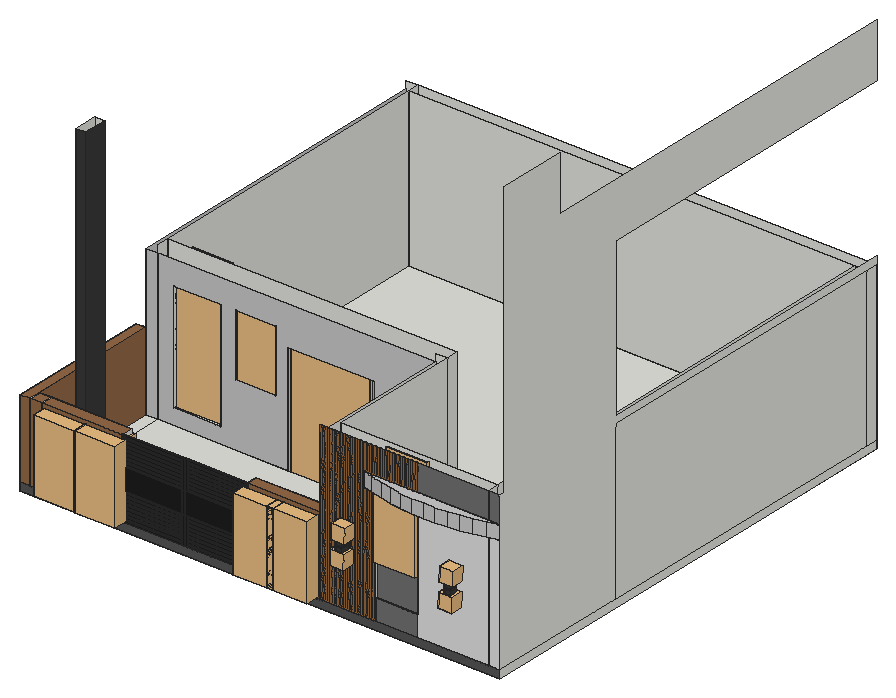
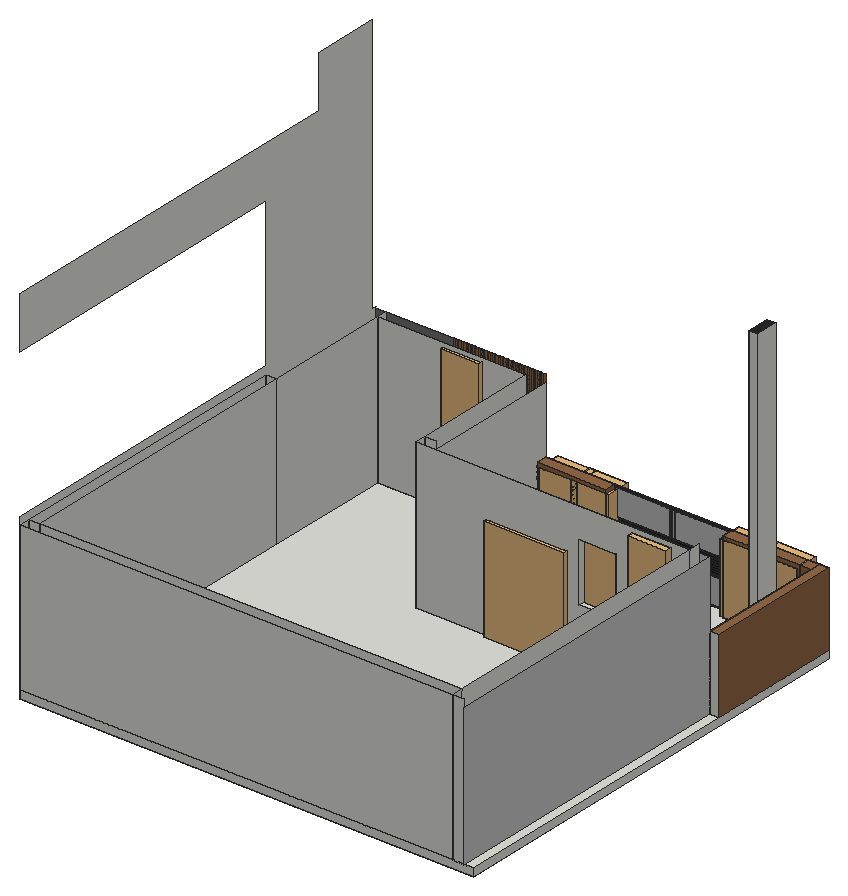
# SketchUp Ruby script. Lengths in inches.
U = 1.inch
M = Sketchup.active_model
def pt(a) = Geom::Point3d.new(a.map { |v| v * U })
def face(e, loops, mat)
  f = e.add_face(loops[0].map { |a| pt(a) })
  loops[1..].each { |l| e.add_face(l.map { |a| pt(a) }).erase! }
  f.material = f.back_material = mat if mat
  f
end
# faces: each face lists its corners as indices into pts; further lists are holes
def faces(e, pts, list, mat = nil) = list.each { |f| face(e, (f[0].is_a?(Array) ? f : [f]).map { |l| l.map { |i| pts[i] } }, mat) }
# xy, xz, yz: faces in a plane at the given z, y or x. An outline is a flat list of corners, or four numbers for a rectangle; further outlines are holes
def ring(l) = l.size == 4 ? [[l[0], l[1]], [l[2], l[1]], [l[2], l[3]], [l[0], l[3]]] : l.each_slice(2).to_a
def flat(e, list, mat, &to3) = list.each { |f| face(e, (f[0].is_a?(Array) ? f : [f]).map { |l| ring(l).map { |u, v| to3.(u, v) } }, mat) }
def xy(e, z, list, mat = nil) = flat(e, list, mat) { |x, y| [x, y, z] }
def xz(e, y, list, mat = nil) = flat(e, list, mat) { |x, z| [x, y, z] }
def yz(e, x, list, mat = nil) = flat(e, list, mat) { |y, z| [x, y, z] }
def lines(e, pts, list) = list.each { |a, b| e.add_line(pt(pts[a]), pt(pts[b])) }
# prism: a flat outline (further loops are holes) pulled along v
def prism(e, loops, v, mat = nil)
  f = face(e, loops, mat); d = Geom::Vector3d.new(v.map { |x| x * U })
  f.pushpull(f.normal.samedirection?(d) ? d.length : -d.length)
end
def box(e, o, s, mat = nil) = prism(e, [[o, [o[0] + s[0], o[1], o[2]], [o[0] + s[0], o[1] + s[1], o[2]], [o[0], o[1] + s[1], o[2]]]], [0, 0, s[2]], mat)
def at(x, y, z, deg = 0) = Geom::Transformation.translation(pt([x, y, z])) * Geom::Transformation.rotation(ORIGIN, Z_AXIS, deg.degrees)
def axes(o, x, y, z) = Geom::Transformation.new([*x, 0, *y, 0, *z, 0, *pt(o).to_a, 1])
def part(name) = M.definitions.add(name)
# library, detail: a bought-in or finely detailed component or shape, given as its bounding box
def library(name, o, s) = part(name).tap { |d| box(d.entities, o, s) }
def detail(e, o, s) = box(e.add_group.entities, o, s)
def put(e, d, t, mat = nil) = e.add_instance(d, t).tap { |i| i.material = mat if mat }
def group(e, t, mat = nil) = e.add_group.tap { |g| g.transformation = t; g.material = mat if mat }.entities
root = M.entities
M.materials.add("11.free-metal-textures").color = [58, 58, 58]
M.materials.add("Color_008").color = [30, 30, 30]
M.materials.add("[0055_LightGoldenrodYellow]").color = [250, 250, 210]
M.materials.add("[0111_SlateGray]1").color = [112, 128, 144]
M.materials.add("[0117_GhostWhite]").color = [248, 248, 255]
M.materials.add("[0131_Silver]1").color = [192, 192, 192]
M.materials.add("[0134_DimGray]").color = [105, 105, 105]
M.materials.add("[Brick Antique 01]").color = [147, 105, 71]
M.materials.add("[Cladding Stucco White]").color = [200, 200, 200]
M.materials.add("[Color M01]").color = [226, 226, 226]
M.materials.add("[Color M05]").color = [114, 114, 114]
M.materials.add("[Color M06]").color = [86, 86, 86]
M.materials.add("[Color M07]").color = [58, 58, 58]
M.materials.add("[Wood Floor]").color = [155, 105, 61]
M.materials.add("images").color = [124, 124, 124]
c1 = library("Door 243 053",[-21.6,-2.79,-0.07],[43.2,5.58,82.64])
c2 = part("Gate slat")
box(c2.entities,[0,0,-2.03],[1.97,0.97,40.94])
c3 = part("Gate frame upright")
box(c3.entities,[0,0,0],[1.9,0.97,93.54])
c4 = part("Gate slat \#1")
box(c4.entities,[2.95,0,-2.03],[0.99,0.97,40.94])
c5 = part("Slatted gate panel")
p = [[42.85,0.97,43.31],[42.85,0.97,44.29]]
lines(c5.entities,p,[[0,1]])
put(c5.entities,c2,axes([3.9375,0,86.61],[0,0,-1],[0,1,0],[1,0,0]),"Color_008")
put(c5.entities,c3,axes([87.6,0,0],[1,0,0],[0,1,0],[0,0,0.92593]),"Color_008")
put(c5.entities,c2,axes([48.6875,0,86.61],[0,0,-1],[0,1,0],[1,0,0]),"Color_008")
put(c5.entities,c3,axes([0,0,0],[1,0,0],[0,1,0],[0,0,0.92593]),"Color_008")
put(c5.entities,c3,axes([42.85,0,0],[1,0,0],[0,1,0],[0,0,0.92593]),"Color_008")
put(c5.entities,c3,axes([44.75,0,0],[1,0,0],[0,1,0],[0,0,0.92593]),"Color_008")
put(c5.entities,c4,axes([3.9375,0,87.11],[0,0,-1],[0,1,0],[1,0,0]),"[0134_DimGray]")
put(c5.entities,c4,axes([48.6875,0,87.11],[0,0,-1],[0,1,0],[1,0,0]),"[0134_DimGray]")
put(c5.entities,c2,axes([48.6875,0,82.68],[0,0,-1],[0,1,0],[1,0,0]),"Color_008")
put(c5.entities,c4,axes([48.6875,0,83.17],[0,0,-1],[0,1,0],[1,0,0]),"[0134_DimGray]")
put(c5.entities,c4,axes([3.9375,0,83.17],[0,0,-1],[0,1,0],[1,0,0]),"[0134_DimGray]")
put(c5.entities,c2,axes([3.9375,0,82.68],[0,0,-1],[0,1,0],[1,0,0]),"Color_008")
put(c5.entities,c4,axes([48.6875,0,75.3],[0,0,-1],[0,1,0],[1,0,0]),"[0134_DimGray]")
put(c5.entities,c2,axes([48.6875,0,78.74],[0,0,-1],[0,1,0],[1,0,0]),"Color_008")
put(c5.entities,c2,axes([48.6875,0,74.8],[0,0,-1],[0,1,0],[1,0,0]),"Color_008")
put(c5.entities,c4,axes([48.6875,0,79.23],[0,0,-1],[0,1,0],[1,0,0]),"[0134_DimGray]")
put(c5.entities,c4,axes([3.9375,0,75.3],[0,0,-1],[0,1,0],[1,0,0]),"[0134_DimGray]")
put(c5.entities,c2,axes([3.9375,0,78.74],[0,0,-1],[0,1,0],[1,0,0]),"Color_008")
put(c5.entities,c4,axes([3.9375,0,79.23],[0,0,-1],[0,1,0],[1,0,0]),"[0134_DimGray]")
put(c5.entities,c2,axes([3.9375,0,74.8],[0,0,-1],[0,1,0],[1,0,0]),"Color_008")
put(c5.entities,c4,axes([48.6875,0,67.42],[0,0,-1],[0,1,0],[1,0,0]),"[0134_DimGray]")
put(c5.entities,c4,axes([3.9375,0,63.48],[0,0,-1],[0,1,0],[1,0,0]),"[0134_DimGray]")
put(c5.entities,c4,axes([48.6875,0,71.36],[0,0,-1],[0,1,0],[1,0,0]),"[0134_DimGray]")
put(c5.entities,c4,axes([3.9375,0,67.42],[0,0,-1],[0,1,0],[1,0,0]),"[0134_DimGray]")
put(c5.entities,c2,axes([3.9375,0,70.87],[0,0,-1],[0,1,0],[1,0,0]),"Color_008")
put(c5.entities,c2,axes([48.6875,0,70.87],[0,0,-1],[0,1,0],[1,0,0]),"Color_008")
put(c5.entities,c2,axes([48.6875,0,66.93],[0,0,-1],[0,1,0],[1,0,0]),"Color_008")
put(c5.entities,c2,axes([48.6875,0,59.06],[0,0,-1],[0,1,0],[1,0,0]),"Color_008")
put(c5.entities,c2,axes([3.9375,0,55.12],[0,0,-1],[0,1,0],[1,0,0]),"Color_008")
put(c5.entities,c2,axes([3.9375,0,62.99],[0,0,-1],[0,1,0],[1,0,0]),"Color_008")
put(c5.entities,c4,axes([3.9375,0,59.55],[0,0,-1],[0,1,0],[1,0,0]),"[0134_DimGray]")
put(c5.entities,c2,axes([3.9375,0,66.93],[0,0,-1],[0,1,0],[1,0,0]),"Color_008")
put(c5.entities,c2,axes([48.6875,0,62.99],[0,0,-1],[0,1,0],[1,0,0]),"Color_008")
put(c5.entities,c4,axes([48.6875,0,59.55],[0,0,-1],[0,1,0],[1,0,0]),"[0134_DimGray]")
put(c5.entities,c4,axes([48.6875,0,63.48],[0,0,-1],[0,1,0],[1,0,0]),"[0134_DimGray]")
put(c5.entities,c2,axes([3.9375,0,59.06],[0,0,-1],[0,1,0],[1,0,0]),"Color_008")
put(c5.entities,c4,axes([3.9375,0,71.36],[0,0,-1],[0,1,0],[1,0,0]),"[0134_DimGray]")
put(c5.entities,c4,axes([3.9375,0,33.96],[0,0,-1],[0,1,0],[1,0,0]),"[0134_DimGray]")
put(c5.entities,c4,axes([48.6875,0,33.96],[0,0,-1],[0,1,0],[1,0,0]),"[0134_DimGray]")
put(c5.entities,c2,axes([3.9375,0,29.53],[0,0,-1],[0,1,0],[1,0,0]),"Color_008")
put(c5.entities,c4,axes([3.9375,0,26.08],[0,0,-1],[0,1,0],[1,0,0]),"[0134_DimGray]")
put(c5.entities,c2,axes([3.9375,0,33.46],[0,0,-1],[0,1,0],[1,0,0]),"Color_008")
put(c5.entities,c2,axes([48.6875,0,29.53],[0,0,-1],[0,1,0],[1,0,0]),"Color_008")
put(c5.entities,c4,axes([48.6875,0,30.02],[0,0,-1],[0,1,0],[1,0,0]),"[0134_DimGray]")
put(c5.entities,c2,axes([3.9375,0,25.59],[0,0,-1],[0,1,0],[1,0,0]),"Color_008")
put(c5.entities,c2,axes([48.6875,0,25.59],[0,0,-1],[0,1,0],[1,0,0]),"Color_008")
put(c5.entities,c2,axes([48.6875,0,33.46],[0,0,-1],[0,1,0],[1,0,0]),"Color_008")
put(c5.entities,c2,axes([3.9375,0,49.7],[0,0,-1],[0,1,0],[1,0,0]),"Color_008")
put(c5.entities,c4,axes([48.6875,0,26.08],[0,0,-1],[0,1,0],[1,0,0]),"[0134_DimGray]")
put(c5.entities,c4,axes([3.9375,0,30.02],[0,0,-1],[0,1,0],[1,0,0]),"[0134_DimGray]")
put(c5.entities,c2,axes([3.9375,0,5.91],[0,0,-1],[0,1,0],[1,0,0]),"Color_008")
put(c5.entities,c2,axes([48.6875,0,13.78],[0,0,-1],[0,1,0],[1,0,0]),"Color_008")
put(c5.entities,c4,axes([48.6875,0,10.33],[0,0,-1],[0,1,0],[1,0,0]),"[0134_DimGray]")
put(c5.entities,c4,axes([3.9375,0,6.4],[0,0,-1],[0,1,0],[1,0,0]),"[0134_DimGray]")
put(c5.entities,c2,axes([3.9375,0,13.78],[0,0,-1],[0,1,0],[1,0,0]),"Color_008")
put(c5.entities,c2,axes([48.6875,0,21.65],[0,0,-1],[0,1,0],[1,0,0]),"Color_008")
put(c5.entities,c2,axes([48.6875,0,5.91],[0,0,-1],[0,1,0],[1,0,0]),"Color_008")
put(c5.entities,c4,axes([48.6875,0,22.15],[0,0,-1],[0,1,0],[1,0,0]),"[0134_DimGray]")
put(c5.entities,c2,axes([48.6875,0,1.97],[0,0,-1],[0,1,0],[1,0,0]),"Color_008")
put(c5.entities,c2,axes([48.6875,0,9.84],[0,0,-1],[0,1,0],[1,0,0]),"Color_008")
put(c5.entities,c4,axes([48.6875,0,6.4],[0,0,-1],[0,1,0],[1,0,0]),"[0134_DimGray]")
put(c5.entities,c2,axes([3.9375,0,9.84],[0,0,-1],[0,1,0],[1,0,0]),"Color_008")
put(c5.entities,c4,axes([3.9375,0,10.33],[0,0,-1],[0,1,0],[1,0,0]),"[0134_DimGray]")
put(c5.entities,c4,axes([3.9375,0,22.15],[0,0,-1],[0,1,0],[1,0,0]),"[0134_DimGray]")
put(c5.entities,c2,axes([3.9375,0,1.97],[0,0,-1],[0,1,0],[1,0,0]),"Color_008")
put(c5.entities,c4,axes([3.9375,0,18.21],[0,0,-1],[0,1,0],[1,0,0]),"[0134_DimGray]")
put(c5.entities,c4,axes([3.9375,0,14.27],[0,0,-1],[0,1,0],[1,0,0]),"[0134_DimGray]")
put(c5.entities,c2,axes([3.9375,0,21.65],[0,0,-1],[0,1,0],[1,0,0]),"Color_008")
put(c5.entities,c4,axes([48.6875,0,18.21],[0,0,-1],[0,1,0],[1,0,0]),"[0134_DimGray]")
put(c5.entities,c2,axes([3.9375,0,17.72],[0,0,-1],[0,1,0],[1,0,0]),"Color_008")
put(c5.entities,c2,axes([48.6875,0,17.72],[0,0,-1],[0,1,0],[1,0,0]),"Color_008")
put(c5.entities,c4,axes([48.6875,0,14.27],[0,0,-1],[0,1,0],[1,0,0]),"[0134_DimGray]")
put(c5.entities,c2,axes([3.9375,0,44.29],[0,0,-1],[0,1,0],[1,0,0]),"Color_008")
put(c5.entities,c2,axes([3.9375,0,38.88],[0,0,-1],[0,1,0],[1,0,0]),"Color_008")
put(c5.entities,c2,axes([48.6875,0,49.7],[0,0,-1],[0,1,0],[1,0,0]),"Color_008")
put(c5.entities,c2,axes([48.6875,0,44.29],[0,0,-1],[0,1,0],[1,0,0]),"Color_008")
put(c5.entities,c2,axes([48.6875,0,38.88],[0,0,-1],[0,1,0],[1,0,0]),"Color_008")
put(c5.entities,c2,axes([48.6875,0,55.12],[0,0,-1],[0,1,0],[1,0,0]),"Color_008")
c6 = part("Gate infill panel \#1")
box(c6.entities,[0,0,-1.97],[52.81,0.39,23.62])
c7 = part("Gate infill panel")
box(c7.entities,[0,0,-9.84],[39.64,0.39,36.58])
c8 = part("Porton casa")
put(c8.entities,c5,axes([13.02,-50.18,0],[0.96774,0,0],[0,1,0],[0,0,1]),"[0055_LightGoldenrodYellow]")
put(c8.entities,c6,axes([13.02,-50.57,33.46],[0.82011,0,0],[0,1,0],[0,0,1]),"Color_008")
put(c8.entities,c7,axes([56.33,-49.21,63.0625],[1.04618,0,0],[0,1,0],[0,0,0.8072]),"[0131_Silver]1")
put(c8.entities,c7,axes([56.33,-49.21,9.91],[1.04618,0,0],[0,1,0],[0,0,0.8072]),"[0131_Silver]1")
put(c8.entities,c7,axes([14.87,-49.21,9.91],[1.04618,0,0],[0,1,0],[0,0,0.8072]),"[0131_Silver]1")
put(c8.entities,c7,axes([14.87,-49.21,63.0625],[1.04618,0,0],[0,1,0],[0,0,0.8072]),"[0131_Silver]1")
put(c8.entities,c6,axes([56.33,-50.57,33.46],[0.82011,0,0],[0,1,0],[0,0,1]),"Color_008")
c9 = library("Curtains 004",[-15.59,-2.26,0],[31.18,4.52,116.91])
c10 = library("Kube Single Down Facing wall light",[-12.125,-6.92,-52.21],[30.76,19.64,56.07])
c11 = library("glass door",[0,-2.95,0],[39.37,5.9,82.68])
c12 = library("Spot Light\#1",[-5.1,-5.1,-11.05],[10.2,10.2,11.05])
c13 = part("Group0\#1")
p = [[-17.97,0.98,0],[-6.48,-16.79,0],[0,0,38],[13.97,-11.35,0],[15.11,9.78,0],[-4.625,17.4,0]]
faces(c13.entities,p,[[0,1,2],[1,3,2],[3,4,2],[5,0,2],[4,5,2]])
c14 = part("Group\#3")
xy(c14.entities,0.16,[[[0,0,5.28,5.28],[0.33,0.33,4.95,4.95]]],"images")
xy(c14.entities,0.6875,[[[0.33,0.33,4.95,4.95],[0.49,0.49,4.78,4.78]]],"[0111_SlateGray]1")
xy(c14.entities,1.48,[[0.49,0.49,4.78,4.78]],"[0117_GhostWhite]")
xy(c14.entities,3.85,[[1.58,9.23,3.69,9.5]],"images")
xy(c14.entities,4.52,[[2.25,5.28,3.03,9.23]],"images")
xy(c14.entities,5.17,[[0,0,5.28,0,5.28,5.28,4.95,5.28,4.95,0.33,0.33,0.33,0.33,5.28,0,5.28],[0.33,4.95,4.95,5.28]])
xy(c14.entities,5.69,[[2.25,6.45,3.03,8.06]])
xy(c14.entities,5.7,[[0,0,0,5.28,0.33,5.28,0.33,0.33,4.95,0.33,4.95,5.28,5.28,5.28,5.28,0]])
xy(c14.entities,6.23,[[0,0,5.28,0,5.28,5.28,4.95,5.28,4.95,0.33,0.33,0.33,0.33,5.28,0,5.28],[2.25,6.45,3.03,8.06]])
xy(c14.entities,6.75,[[0,0,5.28,0,5.28,5.28,4.95,5.28,4.95,0.33,0,0.33],[0,0.33,0.33,5.28],[0.33,4.95,4.95,5.28]])
xy(c14.entities,7.41,[[2.25,5.28,3.03,9.23]],"images")
xy(c14.entities,8.07,[[1.58,9.23,3.69,9.5]],"images")
xy(c14.entities,10.45,[[0.49,0.49,4.78,4.78]],"[0117_GhostWhite]")
xy(c14.entities,11.24,[[[0.33,0.33,4.95,4.95],[0.49,0.49,4.78,4.78]]],"[0111_SlateGray]1")
xy(c14.entities,11.77,[[[0,0,5.28,5.28],[0.33,0.33,4.95,4.95]]],"images")
xz(c14.entities,0,[[0,0.16,5.28,5.17],[0,5.7,5.28,6.23],[0,6.75,5.28,11.77]],"11.free-metal-textures")
xz(c14.entities,0.33,[[0.33,5.7,4.95,5.96],[0.33,5.96,4.95,6.23]])
xz(c14.entities,0.33,[[0.33,0.16,4.95,0.6875],[0.33,11.24,4.95,11.77]],"[0111_SlateGray]1")
xz(c14.entities,0.33,[[0.33,5.17,4.95,5.7],[0.33,6.23,4.95,6.75]],"[0117_GhostWhite]")
xz(c14.entities,0.49,[[0.49,0.6875,4.78,1.48],[0.49,1.48,4.78,10.45],[0.49,10.45,4.78,11.24]],"[0111_SlateGray]1")
xz(c14.entities,4.78,[[0.49,0.6875,4.78,1.48],[0.49,1.48,4.78,10.45],[0.49,10.45,4.78,11.24]],"[0111_SlateGray]1")
xz(c14.entities,4.95,[[0.33,0.16,4.95,0.6875],[0.33,11.24,4.95,11.77]],"[0111_SlateGray]1")
xz(c14.entities,5.28,[[2.25,4.52,3.03,5.17],[2.25,5.17,2.64,6.75],[2.64,5.17,3.03,6.75],[2.25,6.75,3.03,7.41]])
xz(c14.entities,5.28,[[0,0.16,0,5.17,2.25,5.17,2.25,4.52,3.03,4.52,3.03,5.17,5.28,5.17,5.28,0.16],[0.33,5.17,0.33,5.7,0,5.7,0,6.23,0.33,6.23,0.33,6.75,2.25,6.75,2.25,5.17],[3.03,5.17,3.03,6.75,4.95,6.75,4.95,6.23,5.28,6.23,5.28,5.7,4.95,5.7,4.95,5.17],[0,6.75,0,11.77,5.28,11.77,5.28,6.75,3.03,6.75,3.03,7.41,2.25,7.41,2.25,6.75]],"11.free-metal-textures")
xz(c14.entities,6.45,[[2.25,5.69,3.03,6.23]])
xz(c14.entities,8.06,[[2.25,5.69,3.03,6.23]])
xz(c14.entities,9.23,[[1.58,3.85,3.03,3.85,3.03,4.52,2.25,4.52,2.25,7.41,3.03,7.41,3.03,3.85,3.69,3.85,3.69,8.07,1.58,8.07]],"images")
xz(c14.entities,9.5,[[1.58,3.85,3.69,8.07]])
yz(c14.entities,0,[[0,0.16,5.28,5.17],[0,5.7,5.28,6.23],[0,6.75,5.28,11.77]],"11.free-metal-textures")
yz(c14.entities,0.33,[[0.33,5.7,4.95,5.96]])
yz(c14.entities,0.33,[[0.33,0.16,4.95,0.6875],[0.33,11.24,4.95,11.77]],"[0111_SlateGray]1")
yz(c14.entities,0.33,[[0.33,5.17,5.28,5.7],[0.33,6.23,5.28,6.75]],"[0117_GhostWhite]")
yz(c14.entities,0.49,[[0.49,0.6875,4.78,1.48],[0.49,1.48,4.78,10.45],[0.49,10.45,4.78,11.24]],"[0111_SlateGray]1")
yz(c14.entities,1.58,[[9.23,3.85,9.5,8.07]],"images")
yz(c14.entities,2.25,[[[5.28,4.52,9.23,7.41],[6.45,5.69,8.06,6.23]]],"images")
yz(c14.entities,3.03,[[[5.28,4.52,9.23,7.41],[6.45,5.69,8.06,6.23]]],"images")
yz(c14.entities,3.69,[[9.23,3.85,9.5,8.07]],"images")
yz(c14.entities,4.78,[[0.49,0.6875,4.78,1.48],[0.49,1.48,4.78,10.45],[0.49,10.45,4.78,11.24]],"[0111_SlateGray]1")
yz(c14.entities,4.95,[[0.33,5.7,4.95,5.96]])
yz(c14.entities,4.95,[[0.33,0.16,4.95,0.6875],[0.33,11.24,4.95,11.77]],"[0111_SlateGray]1")
yz(c14.entities,4.95,[[0.33,5.17,5.28,5.7],[0.33,6.23,5.28,6.75]],"[0117_GhostWhite]")
yz(c14.entities,5.28,[[0,0.16,5.28,5.17],[0,5.7,5.28,6.23],[0,6.75,5.28,11.77]],"11.free-metal-textures")
p = [[4.95,4.95,5.96],[0.33,4.95,5.96],[3.03,5.28,4.38],[3.03,5.28,4.52],[3.03,9.23,3.73],[3.03,9.23,3.85]]
lines(c14.entities,p,[[0,1],[2,3],[4,5]])
put(c14.entities,c13,axes([2.51,2.87,0],[0.10834,0,0],[0,0.10834,0],[0,0,0.10834]))
put(c14.entities,c13,axes([2.78,2.43,12.06],[-0.10834,0,0],[0,0.10834,0],[0,0,-0.10834]))
c15 = library("Window 46-05",[-17.86,-2.78,0],[35.72,4.26,58.96])
xy(root,-6,[[0.25,25,367.875,385]])
xy(root,0,[[0.25,25,7.875,136],[7.875,25,16.875,34],[16.875,25,78.59,34],[[78.59,25,173.68,25,173.68,34,229.875,34,229.875,136,178.875,136,178.875,145,118.875,145,118.875,136,16.875,136,16.875,34,78.59,34],[23.52,49.11,30.9,67.43]],[173.68,25,229.875,34],
  [229.875,25,238.875,136],[238.875,25,358.875,34],[358.875,25,367.875,136],[7.875,34,16.875,136],[238.875,34,358.875,34,358.875,376,16.875,376,16.875,145,238.875,145],
  [0.25,136,7.875,385],[7.875,136,16.875,385],[16.875,136,118.875,145],[178.875,136,238.875,145],[178.875,136,238.875,145],
  [358.875,136,367.875,376],[16.875,376,367.875,385]])
xy(root,12,[[28.875,136,64.875,145]])
xy(root,15.97,[[272.51,25,304.7,26]])
xy(root,41.9,[[272.51,25,304.7,26]])
xy(root,43.2,[[273.0625,25,304.625,34]])
xy(root,48,[[76.875,136,106.875,145]])
xy(root,60,[[0.25,25,7.875,136],[7.875,25,16.875,34],[16.875,25,78.59,34],[173.68,25,229.875,34]],"[Brick Antique 01]")
xy(root,84,[[118.875,136,178.875,145]])
xy(root,89.01,[[273.0625,25,304.625,34]])
xy(root,89.3125,[[315.625,16.6875,306.77,16.92,297.95,17.62,289.17,18.78,280.47,20.4,271.86,22.47,263.375,25,367.875,25,359.39,22.47,350.78,20.4,342.08,18.78,333.3,17.62,324.48,16.92]])
xy(root,96,[[28.875,136,64.875,145],[76.875,136,106.875,145]])
xy(root,99.8125,[[315.625,16.6875,324.48,16.92,333.3,17.62,342.08,18.78,350.78,20.4,359.39,22.47,367.875,25,263.375,25,271.86,22.47,280.47,20.4,289.17,18.78,297.95,17.62,306.77,16.92]],"[Cladding Stucco White]")
xz(root,25,[[263.375,89.3125,264.5625,99.8125],[264.5625,89.3125,266,99.8125],[266,89.3125,267.1875,99.8125],[267.1875,89.3125,268.625,99.8125],[268.625,89.3125,269.8125,99.8125],
  [269.8125,89.3125,358.875,99.8125],[358.875,89.3125,367.875,99.8125]])
xz(root,25,[[0.25,0,7.875,60],[7.875,0,16.875,60],[16.875,0,78.59,60],[173.68,0,229.875,60]],"[Brick Antique 01]")
xz(root,25,[[[272.375,0,272.51,0,272.51,41.9,304.7,41.9,304.7,0,358.875,0,358.875,89.3125,272.375,89.3125],[273.0625,43.2,304.625,89.01]],[358.875,0,367.875,89.3125]],"[Color M01]")
xz(root,25,[[272.51,0,304.7,15.97],[304.7,99.8125,358.875,120],[358.875,99.8125,367.875,120]],"[Color M05]")
xz(root,25,[[0.25,-6,367.875,0]],"[Color M06]")
xz(root,25,[[229.875,0,231.0625,120],[231.0625,0,232.4375,120],[232.4375,0,233.625,120],[233.625,0,235,120],[235,0,236.1875,120],
  [236.1875,0,237.5625,120],[237.5625,0,238.75,120],[238.75,0,240.125,120],[240.125,0,241.3125,120],[241.3125,0,242.6875,120],
  [242.6875,0,243.875,120],[243.875,0,245.25,120],[245.25,0,246.4375,120],[246.4375,0,247.8125,120],[247.8125,0,249,120],
  [249,0,250.375,120],[250.375,0,251.5625,120],[251.5625,0,252.9375,120],[252.9375,0,254.125,120],[254.125,0,255.5,120],
  [255.5,0,256.6875,120],[256.6875,0,258.125,120],[258.125,0,259.3125,120],[259.3125,0,260.75,120],[260.75,0,261.9375,120],
  [261.9375,0,263.375,120],[263.375,0,264.5625,89.3125],[264.5625,0,266,89.3125],[266,0,267.1875,89.3125],[267.1875,0,268.625,89.3125],
  [268.625,0,269.8125,89.3125],[269.8125,0,271.1875,89.3125],[271.1875,0,272.375,89.3125],[263.375,99.8125,264.5625,120],[264.5625,99.8125,266,120],
  [266,99.8125,267.1875,120],[267.1875,99.8125,268.625,120],[268.625,99.8125,269.8125,120],[269.8125,99.8125,271.125,120],[271.125,99.8125,272.3125,120],
  [272.3125,99.8125,273.625,120],[273.625,99.8125,274.8125,120],[274.8125,99.8125,276.125,120],[276.125,99.8125,277.3125,120],[277.3125,99.8125,278.625,120],
  [278.625,99.8125,279.8125,120],[279.8125,99.8125,281.125,120],[281.125,99.8125,282.3125,120],[282.3125,99.8125,283.625,120],[283.625,99.8125,284.8125,120],
  [284.8125,99.8125,286.125,120],[286.125,99.8125,287.3125,120],[287.3125,99.8125,288.625,120],[288.625,99.8125,289.8125,120],[289.8125,99.8125,291.125,120],
  [291.125,99.8125,292.3125,120],[292.3125,99.8125,293.625,120],[293.625,99.8125,294.8125,120],[294.8125,99.8125,296.125,120],[296.125,99.8125,297.3125,120],
  [297.3125,99.8125,298.6875,120],[298.6875,99.8125,299.875,120],[299.875,99.8125,301.25,120],[301.25,99.8125,302.4375,120],[302.4375,99.8125,303.8125,120],
  [303.8125,99.8125,304.7,120]],"[Wood Floor]")
xz(root,26,[[272.51,15.97,304.7,41.9]],"[Color M05]")
xz(root,34,[[[238.875,0,358.875,120],[273.0625,43.2,304.625,89.01]]])
xz(root,34,[[7.875,0,16.875,60],[16.875,0,78.59,60],[173.68,0,229.875,60]],"[Brick Antique 01]")
xz(root,49.11,[[23.52,0,30.9,240]],"[Color M07]")
xz(root,67.43,[[23.52,0,30.9,240]])
xz(root,136,[[0.25,0,7.875,60],[229.875,0,238.875,120],[358.875,0,367.875,120]])
xz(root,136,[[7.875,0,16.875,114],[[16.875,0,118.875,0,118.875,84,178.875,84,178.875,0,229.875,0,229.875,114,16.875,114],[28.875,12,64.875,96],[76.875,48,106.875,96]]],"[Cladding Stucco White]")
xz(root,145,[[[16.875,0,16.875,120,238.875,120,238.875,0,178.875,0,178.875,84,118.875,84,118.875,0],[28.875,12,64.875,96],[76.875,48,106.875,96]]])
xz(root,376,[[16.875,0,358.875,120],[358.875,0,367.875,120]])
xz(root,385,[[0.25,-6,367.875,0],[7.875,0,16.875,120],[16.875,0,367.875,120]])
yz(root,0.25,[[25,-6,385,0]])
yz(root,0.25,[[25,0,136,60]],"[Brick Antique 01]")
yz(root,7.875,[[25,0,34,60]])
yz(root,7.875,[[34,0,136,60]],"[Brick Antique 01]")
yz(root,7.875,[[136,0,385,114]],"[Cladding Stucco White]")
yz(root,16.875,[[25,0,34,60],[136,0,145,120],[145,0,376,120],[376,0,385,120]])
yz(root,23.52,[[49.11,0,67.43,240]])
yz(root,28.875,[[136,12,145,96]])
yz(root,30.9,[[49.11,0,67.43,240]],"[Color M07]")
yz(root,64.875,[[136,12,145,96]])
yz(root,76.875,[[136,48,145,96]])
yz(root,78.59,[[25,0,34,60]])
yz(root,106.875,[[136,48,145,96]])
yz(root,118.875,[[136,0,145,84]])
yz(root,173.68,[[25,0,34,60]],"[Brick Antique 01]")
yz(root,178.875,[[136,0,145,84]])
yz(root,229.875,[[25,0,34,60],[34,0,34,60,25,60,25,114,136,114,136,0]])
yz(root,238.875,[[34,0,136,120],[136,0,145,120]])
yz(root,272.51,[[25,15.97,26,41.9]])
yz(root,273.0625,[[25,43.2,34,89.01]])
yz(root,304.625,[[25,43.2,34,89.01]])
yz(root,304.7,[[25,15.97,26,41.9]],"[Color M05]")
yz(root,358.875,[[25,0,34,120],[34,0,136,120],[136,0,376,120]])
yz(root,367.875,[[25,-6,385,0],[25,0,136,0,136,120,385,120,385,126,136,126,136,246,385,246,385,288,82.27,288,82.27,330,28.62,330,28.62,120.1875,24,120.1875,24,120,25,120],[136,0,376,120],[376,0,385,120]])
p = [[315.625,16.6875,99.8125],[306.77,16.92,99.8125],[306.77,16.92,89.3125],[315.625,16.6875,89.3125],[324.48,16.92,99.8125],[324.48,16.92,89.3125],
  [297.95,17.62,99.8125],[297.95,17.62,89.3125],[333.3,17.62,99.8125],[333.3,17.62,89.3125],[289.17,18.78,99.8125],[289.17,18.78,89.3125],
  [342.08,18.78,99.8125],[342.08,18.78,89.3125],[280.47,20.4,99.8125],[280.47,20.4,89.3125],[350.78,20.4,99.8125],[350.78,20.4,89.3125],
  [271.86,22.47,99.8125],[271.86,22.47,89.3125],[359.39,22.47,99.8125],[359.39,22.47,89.3125],[263.375,25,99.8125],[263.375,25,89.3125],
  [367.875,25,99.8125],[367.875,25,89.3125]]
faces(root,p,[[0,1,2,3],[4,0,3,5],[1,6,7,2],[8,4,5,9],[6,10,11,7],[12,8,9,13],[10,14,15,11],[16,12,13,17],
  [14,18,19,15],[20,16,17,21],[18,22,23,19],[24,20,21,25]],"[Cladding Stucco White]")
put(root,c1,axes([149.15,141.89,0],[1.5125,0,0],[0,2.11547,0],[0,0,1.01736]))
put(root,c8,axes([63.58,75.18,0],[1.1128,0,0],[0,1,0],[0,0,0.69319]))
put(root,c9,at(46.77,148.75,0))
put(root,c9,at(290.02,34.29,0))
put(root,c10,at(183.19,21.65,53.23))
put(root,c10,at(209.25,21.65,53.23))
put(root,c10,at(62.32,21.65,53.23))
put(root,c10,at(30.75,21.65,53.23))
put(root,c11,axes([28.875,139.93,12],[0.9144,0,0],[0,0.67,0],[0,0,1.016]))
put(root,c12,axes([249.99,20.98,43.58],[-0.99919,0,0.04013],[0,1,0],[0.04013,0,0.99919]))
put(root,c12,axes([333.17,20.98,43.58],[-0.99919,0,0.04013],[0,1,0],[0.04013,0,0.99919]))
put(root,c14,axes([247.47,17.32,52.76],[1,0,0],[0,1,0],[0,0,-1]))
put(root,c14,axes([330.66,17.32,52.76],[1,0,0],[0,1,0],[0,0,-1]))
put(root,c15,axes([288.54,25.24,41.9],[0.90044,0,0],[0,1,0],[0,0,0.79903]))
put(root,c15,axes([92.16,138.85,48],[0.85541,0,0],[0,0.95,0],[0,0,0.82095]))
put(root,c12,axes([250.27,20.98,50.65],[-0.99919,0,0.04013],[0,1,0],[-0.04013,0,-0.99919]))
put(root,c12,axes([333.46,20.98,50.65],[-0.99919,0,0.04013],[0,1,0],[-0.04013,0,-0.99919]))
